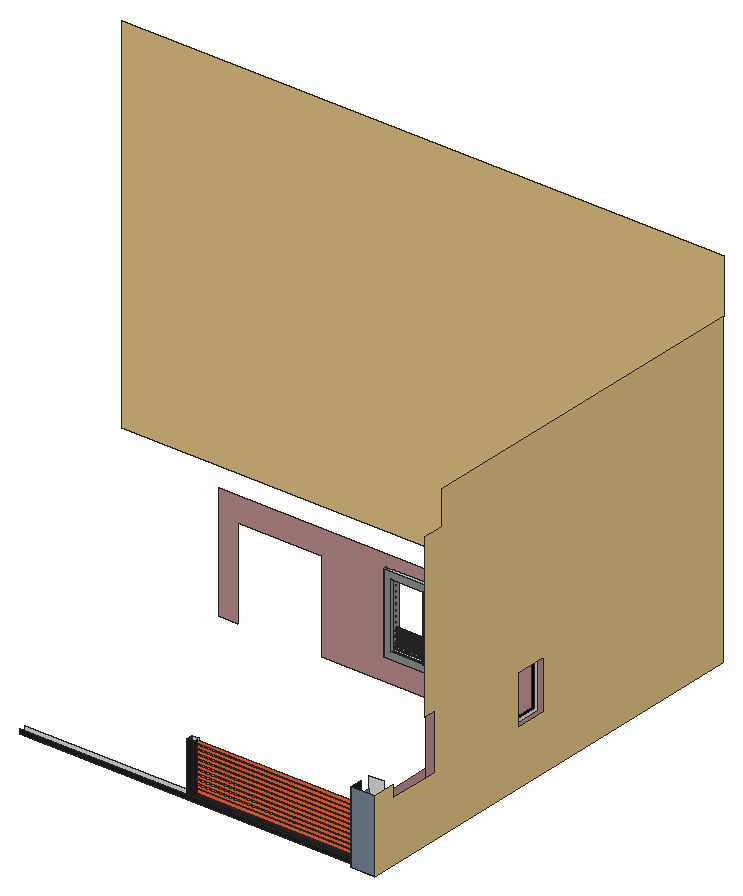
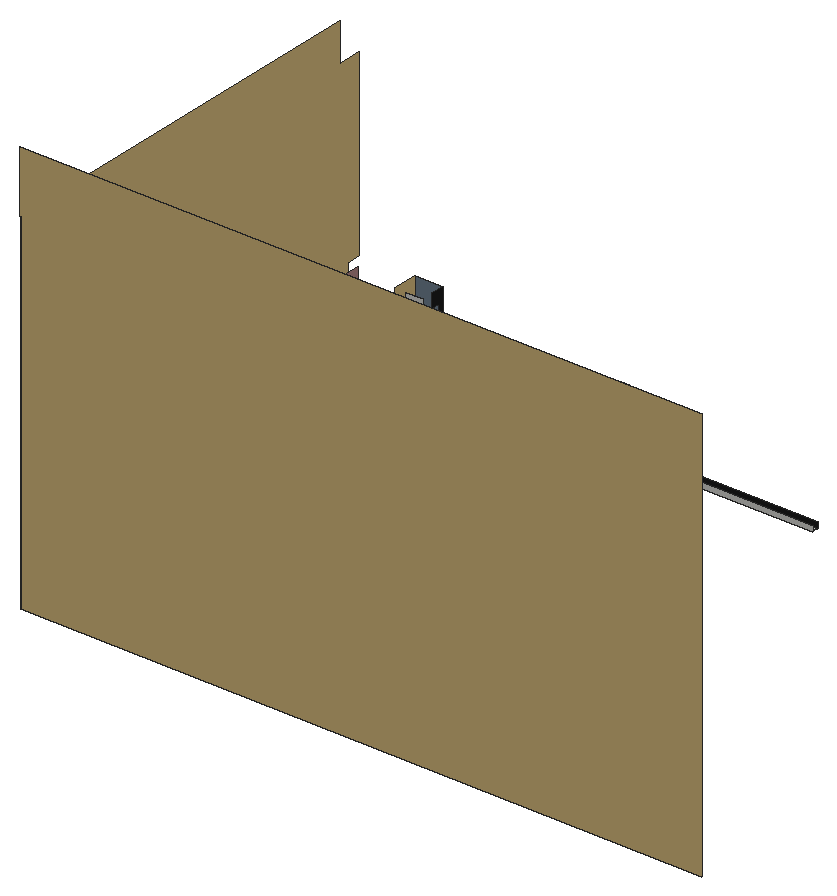
# SketchUp Ruby script. Lengths in inches.
U = 1.inch
M = Sketchup.active_model
def pt(a) = Geom::Point3d.new(a.map { |v| v * U })
def face(e, loops, mat)
  f = e.add_face(loops[0].map { |a| pt(a) })
  loops[1..].each { |l| e.add_face(l.map { |a| pt(a) }).erase! }
  f.material = f.back_material = mat if mat
  f
end
# faces: each face lists its corners as indices into pts; further lists are holes
def faces(e, pts, list, mat = nil) = list.each { |f| face(e, (f[0].is_a?(Array) ? f : [f]).map { |l| l.map { |i| pts[i] } }, mat) }
# xy, xz, yz: faces in a plane at the given z, y or x. An outline is a flat list of corners, or four numbers for a rectangle; further outlines are holes
def ring(l) = l.size == 4 ? [[l[0], l[1]], [l[2], l[1]], [l[2], l[3]], [l[0], l[3]]] : l.each_slice(2).to_a
def flat(e, list, mat, &to3) = list.each { |f| face(e, (f[0].is_a?(Array) ? f : [f]).map { |l| ring(l).map { |u, v| to3.(u, v) } }, mat) }
def xy(e, z, list, mat = nil) = flat(e, list, mat) { |x, y| [x, y, z] }
def xz(e, y, list, mat = nil) = flat(e, list, mat) { |x, z| [x, y, z] }
def yz(e, x, list, mat = nil) = flat(e, list, mat) { |y, z| [x, y, z] }
def lines(e, pts, list) = list.each { |a, b| e.add_line(pt(pts[a]), pt(pts[b])) }
# prism: a flat outline (further loops are holes) pulled along v
def prism(e, loops, v, mat = nil)
  f = face(e, loops, mat); d = Geom::Vector3d.new(v.map { |x| x * U })
  f.pushpull(f.normal.samedirection?(d) ? d.length : -d.length)
end
def box(e, o, s, mat = nil) = prism(e, [[o, [o[0] + s[0], o[1], o[2]], [o[0] + s[0], o[1] + s[1], o[2]], [o[0], o[1] + s[1], o[2]]]], [0, 0, s[2]], mat)
def at(x, y, z, deg = 0) = Geom::Transformation.translation(pt([x, y, z])) * Geom::Transformation.rotation(ORIGIN, Z_AXIS, deg.degrees)
def axes(o, x, y, z) = Geom::Transformation.new([*x, 0, *y, 0, *z, 0, *pt(o).to_a, 1])
def part(name) = M.definitions.add(name)
# library, detail: a bought-in or finely detailed component or shape, given as its bounding box
def library(name, o, s) = part(name).tap { |d| box(d.entities, o, s) }
def detail(e, o, s) = box(e.add_group.entities, o, s)
def put(e, d, t, mat = nil) = e.add_instance(d, t).tap { |i| i.material = mat if mat }
def group(e, t, mat = nil) = e.add_group.tap { |g| g.transformation = t; g.material = mat if mat }.entities
root = M.entities
M.materials.add("[0110_LightSlateGray]").color = [119, 136, 153]
M.materials.add("[0119_RosyBrown]").color = [188, 143, 143]
M.materials.add("[Blacktop Old 02]").color = [143, 145, 145]
M.materials.add("[Color B04]").color = [255, 101, 50]
M.materials.add("[Color M08]").color = [30, 30, 30]
M.materials.add("[Color M09]").color = [0, 0, 0]
M.materials.add("[Concrete Aggregate Smoke]").color = [154, 150, 148]
M.materials.add("[Stone Brushed Khaki]").color = [226, 197, 133]
M.materials.add("[Wood Lumber ButtJoined]").color = [164, 152, 112]
xy(root,0,[[587.78,0,587.78,22.38,602.49,22.38,602.49,74.42,612,74.42,612,0],[254.58,3.88,587.78,6.88],[254.58,6.88,587.78,9.88],[603,74.42,612,135.46],[603,135.46,612,145.85]])
xy(root,4.99,[[421.18,3.88,428.27,6.88],[421.18,6.88,428.27,9.88],[428.27,6.88,587.78,9.88]])
xy(root,4.99,[[428.27,3.88,587.78,6.88]],"[Color M08]")
xy(root,5.875,[[428.27,6.88,587.78,9.88]],"[Color B04]")
xy(root,7.15,[[428.27,6.88,587.78,9.88]],"[Color B04]")
xy(root,10.3125,[[428.27,6.88,587.78,9.88]],"[Color B04]")
xy(root,11.59,[[428.27,6.88,587.78,9.88]],"[Color B04]")
xy(root,14.75,[[428.27,6.88,587.78,9.88]],"[Color B04]")
xy(root,16.03,[[428.27,6.88,587.78,9.88]],"[Color B04]")
xy(root,19.1875,[[428.27,6.88,587.78,9.88]],"[Color B04]")
xy(root,20.46,[[428.27,9.82,587.78,9.88],[428.27,9.88,587.78,9.95],[428.27,9.95,587.78,10.01],[428.27,10.01,587.78,10.13]])
xy(root,20.46,[[428.27,6.88,587.78,9.82]],"[Color B04]")
xy(root,23.35,[[425.53,244.17,512.22,247.17]])
xy(root,23.625,[[428.27,9.82,587.78,9.88],[428.27,9.88,587.78,9.95],[428.27,9.95,587.78,10.01],[428.27,10.01,587.78,10.13]])
xy(root,23.625,[[428.27,6.88,587.78,9.82]],"[Color B04]")
xy(root,24.9,[[428.27,6.88,587.78,9.88]],"[Color B04]")
xy(root,28.0625,[[428.27,6.88,587.78,9.88]],"[Color B04]")
xy(root,29.34,[[428.27,6.88,587.78,9.88]],"[Color B04]")
xy(root,30.2,[[432.38,244.17,464.5,247.17],[464.5,244.17,468.88,247.17],[468.88,244.17,505.38,247.17],[432.38,247.17,464.5,254.42],[468.88,247.17,505.38,254.42]])
xy(root,32.5,[[428.27,6.88,587.78,9.88]],"[Color B04]")
xy(root,33.78,[[428.27,6.88,587.78,9.88]],"[Color B04]")
xy(root,36.9375,[[428.27,6.88,587.78,9.88]],"[Color B04]")
xy(root,38.21,[[428.27,9.88,587.78,10.32]])
xy(root,38.21,[[428.27,6.88,587.78,9.88]],"[Color B04]")
xy(root,41.375,[[428.27,9.88,587.78,10.32]])
xy(root,41.375,[[428.27,6.88,587.78,9.88]],"[Color B04]")
xy(root,42.65,[[428.27,6.88,587.78,9.88]],"[Color B04]")
xy(root,45.8125,[[428.27,6.88,587.78,9.88]],"[Color B04]")
xy(root,47.09,[[428.27,6.88,587.78,9.88]],"[Color B04]")
xy(root,50.25,[[428.27,6.88,587.78,9.88]],"[Color B04]")
xy(root,50.59,[[600,174.3,603,214.68]])
xy(root,51.53,[[428.27,6.88,587.78,9.88]],"[Color B04]")
xz(root,0,[[587.78,0,612,72]],"[0110_LightSlateGray]")
xz(root,3.88,[[254.58,0,587.78,4.99],[421.18,4.99,428.27,54.6875]],"[Color M08]")
xz(root,6.88,[[428.27,4.99,587.78,5.875],[428.27,7.15,587.78,10.3125],[428.27,11.59,587.78,14.75],[428.27,16.03,587.78,19.1875],[428.27,20.46,587.78,23.625],
  [428.27,24.9,587.78,28.0625],[428.27,29.34,587.78,32.5],[428.27,33.78,587.78,36.9375],[428.27,38.21,587.78,41.375],[428.27,42.65,587.78,45.8125],
  [428.27,47.09,587.78,50.25],[428.27,51.53,587.78,54.6875]],"[Color B04]")
xz(root,9.82,[[428.27,20.46,587.78,23.625]])
xz(root,9.88,[[254.58,0,254.58,4.99,428.27,4.99,428.27,2.71,587.78,2.71,587.78,1.4375,428.27,1.4375,428.27,0],[428.27,0,587.78,1.4375],[428.27,2.71,587.78,4.99],[421.18,4.99,428.27,54.6875],[428.27,4.99,587.78,5.875],
  [417.81,6.88,420.87,9],[428.27,7.15,587.78,10.3125],[428.27,11.59,587.78,14.75],[428.27,16.03,587.78,19.1875],[428.27,20.46,587.78,23.625],
  [428.27,24.9,587.78,28.0625],[428.27,29.34,587.78,32.5],[428.27,33.78,587.78,36.9375],[428.27,38.21,587.78,41.375],[428.27,42.65,587.78,45.8125],
  [428.27,47.09,587.78,50.25]])
xz(root,9.88,[[428.27,5.875,587.78,7.15],[428.27,10.3125,587.78,11.59],[428.27,14.75,587.78,16.03],[428.27,19.1875,587.78,20.46],[428.27,23.625,587.78,24.9],
  [428.27,28.0625,587.78,29.34],[428.27,32.5,587.78,33.78],[428.27,36.9375,587.78,38.21],[428.27,41.375,587.78,42.65],[428.27,45.8125,587.78,47.09],
  [428.27,50.25,587.78,51.53]],"[Color B04]")
xz(root,9.95,[[428.27,20.46,587.78,23.625]])
xz(root,10.01,[[428.27,20.46,587.78,23.625]])
xz(root,10.13,[[428.27,20.46,587.78,23.625]])
xz(root,10.32,[[428.27,38.21,587.78,41.375]])
xz(root,22.38,[[587.78,0,602.49,72]])
xz(root,74.42,[[602.49,0,603,60]])
xz(root,174.3,[[600,50.59,603,107.78]],"[Color M09]")
xz(root,214.68,[[600,50.59,603,107.78]])
xz(root,244.17,[[[425.53,23.35,512.22,102.79],[432.38,30.2,505.38,95.95]]],"[Blacktop Old 02]")
xz(root,244.17,[[464.5,30.2,468.88,95.95]],"[Concrete Aggregate Smoke]")
xz(root,247.17,[[[425.53,23.35,512.22,102.79],[432.38,30.2,505.38,95.95]]])
xz(root,247.17,[[[258.19,0,276.99,0,276.99,90.23,361.45,90.23,361.45,0,603,0,603,115.0625,566.2,115.0625,566.2,120,557.23,120,557.23,115.0625,515.23,115.0625,515.23,120,511.18,120,511.18,115.0625,473.23,115.0625,473.23,120,464.26,120,464.26,115.0625,258.19,115.0625],[425.53,23.35,512.22,102.79]]],"[0119_RosyBrown]")
xz(root,434.42,[[12,0,12,364.4375,612.4375,364.4375,612.4375,310.0625,612,310.0625,612,0]],"[Stone Brushed Khaki]")
yz(root,420.87,[[6.88,6.88,9.88,9]])
yz(root,421.18,[[6.88,10.58,9.88,12.6875],[6.88,14.45,9.88,16.5625],[6.88,18.26,9.88,20.375],[6.88,22.08,9.88,24.1875],[6.88,25.89,9.88,28],
  [6.88,29.7,9.88,31.8125],[6.88,33.51,9.88,35.625],[6.88,37.33,9.88,39.4375],[6.88,41.14,9.88,43.25],[6.88,44.95,9.88,47.0625],
  [6.88,48.76,9.88,50.875]])
yz(root,421.18,[[3.88,4.99,3.88,54.6875,6.88,54.6875,6.88,52.58,9.88,52.58,9.88,50.875,6.88,50.875,6.88,48.76,9.88,48.76,9.88,47.0625,6.88,47.0625,6.88,44.95,9.88,44.95,9.88,43.25,6.88,43.25,6.88,41.14,9.88,41.14,9.88,39.4375,6.88,39.4375,6.88,37.33,9.88,37.33,9.88,35.625,6.88,35.625,6.88,33.51,9.88,33.51,9.88,31.8125,6.88,31.8125,6.88,29.7,9.88,29.7,9.88,28,6.88,28,6.88,25.89,9.88,25.89,9.88,24.1875,6.88,24.1875,6.88,22.08,9.88,22.08,9.88,20.375,6.88,20.375,6.88,18.26,9.88,18.26,9.88,16.5625,6.88,16.5625,6.88,14.45,9.88,14.45,9.88,12.6875,6.88,12.6875,6.88,10.58,9.88,10.58,9.88,4.99]],"[Color M08]")
yz(root,425.53,[[244.17,23.35,247.17,102.79]],"[Blacktop Old 02]")
yz(root,428.27,[[6.88,4.99,9.88,5.875],[6.88,7.15,9.88,10.3125],[6.88,11.59,9.88,14.75],[6.88,16.03,9.88,19.1875],[6.88,20.46,9.82,23.625],
  [9.82,20.46,9.88,23.625],[9.88,20.46,9.95,23.625],[9.95,20.46,10.01,23.625],[10.01,20.46,10.13,23.625],[6.88,24.9,9.88,28.0625],
  [6.88,29.34,9.88,32.5],[6.88,33.78,9.88,36.9375],[6.88,38.21,9.88,41.375],[9.88,38.21,10.32,41.375],[6.88,42.65,9.88,45.8125],
  [6.88,47.09,9.88,50.25],[6.88,51.53,9.88,54.6875]])
yz(root,428.27,[[3.88,4.99,6.88,4.99,6.88,5.875,9.88,5.875,9.88,7.15,6.88,7.15,6.88,10.3125,9.88,10.3125,9.88,11.59,6.88,11.59,6.88,14.75,9.88,14.75,9.88,16.03,6.88,16.03,6.88,19.1875,9.88,19.1875,9.88,20.46,6.88,20.46,6.88,23.625,9.88,23.625,9.88,24.9,6.88,24.9,6.88,28.0625,9.88,28.0625,9.88,29.34,6.88,29.34,6.88,32.5,9.88,32.5,9.88,33.78,6.88,33.78,6.88,36.9375,9.88,36.9375,9.88,38.21,6.88,38.21,6.88,41.375,9.88,41.375,9.88,42.65,6.88,42.65,6.88,45.8125,9.88,45.8125,9.88,47.09,6.88,47.09,6.88,50.25,9.88,50.25,9.88,51.53,6.88,51.53,6.88,54.6875,3.88,54.6875]],"[Color M08]")
yz(root,432.38,[[244.17,30.2,247.17,95.95],[[247.17,30.2,254.42,95.95],[250.66,85.64,250.21,85.7,249.78,85.88,249.42,86.16,249.14,86.52,248.97,86.94,248.91,87.39,248.97,87.85,249.14,88.27,249.42,88.63,249.78,88.91,250.21,89.09,250.66,89.14,251.11,89.09,251.53,88.91,251.9,88.63,252.18,88.27,252.35,87.85,252.41,87.39,252.35,86.94,252.18,86.52,251.9,86.16,251.53,85.88,251.11,85.7],[250.66,80.08,250.21,80.14,249.78,80.32,249.42,80.59,249.14,80.96,248.97,81.38,248.91,81.83,248.97,82.29,249.14,82.71,249.42,83.07,249.78,83.35,250.21,83.52,250.66,83.58,251.11,83.52,251.53,83.35,251.9,83.07,252.18,82.71,252.35,82.29,252.41,81.83,252.35,81.38,252.18,80.96,251.9,80.59,251.53,80.32,251.11,80.14],[250.66,74.52,250.21,74.58,249.78,74.75,249.42,75.03,249.14,75.39,248.97,75.82,248.91,76.27,248.97,76.72,249.14,77.14,249.42,77.51,249.78,77.79,250.21,77.96,250.66,78.02,251.11,77.96,251.53,77.79,251.9,77.51,252.18,77.14,252.35,76.72,252.41,76.27,252.35,75.82,252.18,75.39,251.9,75.03,251.53,74.75,251.11,74.58],[250.66,68.96,250.21,69.02,249.78,69.19,249.42,69.47,249.14,69.83,248.97,70.25,248.91,70.71,248.97,71.16,249.14,71.58,249.42,71.94,249.78,72.22,250.21,72.4,250.66,72.46,251.11,72.4,251.53,72.22,251.9,71.94,252.18,71.58,252.35,71.16,252.41,70.71,252.35,70.25,252.18,69.83,251.9,69.47,251.53,69.19,251.11,69.02],[250.66,63.39,250.21,63.45,249.78,63.63,249.42,63.91,249.14,64.27,248.97,64.69,248.91,65.14,248.97,65.6,249.14,66.02,249.42,66.38,249.78,66.66,250.21,66.84,250.66,66.89,251.11,66.84,251.53,66.66,251.9,66.38,252.18,66.02,252.35,65.6,252.41,65.14,252.35,64.69,252.18,64.27,251.9,63.91,251.53,63.63,251.11,63.45],[250.66,57.83,250.21,57.89,249.78,58.07,249.42,58.34,249.14,58.71,248.97,59.13,248.91,59.58,248.97,60.04,249.14,60.46,249.42,60.82,249.78,61.1,250.21,61.27,250.66,61.33,251.11,61.27,251.53,61.1,251.9,60.82,252.18,60.46,252.35,60.04,252.41,59.58,252.35,59.13,252.18,58.71,251.9,58.34,251.53,58.07,251.11,57.89],[250.66,52.27,250.21,52.33,249.78,52.5,249.42,52.78,249.14,53.14,248.97,53.57,248.91,54.02,248.97,54.47,249.14,54.89,249.42,55.26,249.78,55.54,250.21,55.71,250.66,55.77,251.11,55.71,251.53,55.54,251.9,55.26,252.18,54.89,252.35,54.47,252.41,54.02,252.35,53.57,252.18,53.14,251.9,52.78,251.53,52.5,251.11,52.33],[250.66,46.71,250.21,46.77,249.78,46.94,249.42,47.22,249.14,47.58,248.97,48,248.91,48.46,248.97,48.91,249.14,49.33,249.42,49.69,249.78,49.97,250.21,50.15,250.66,50.21,251.11,50.15,251.53,49.97,251.9,49.69,252.18,49.33,252.35,48.91,252.41,48.46,252.35,48,252.18,47.58,251.9,47.22,251.53,46.94,251.11,46.77],[250.66,41.14,250.21,41.2,249.78,41.38,249.42,41.66,249.14,42.02,248.97,42.44,248.91,42.89,248.97,43.35,249.14,43.77,249.42,44.13,249.78,44.41,250.21,44.59,250.66,44.64,251.11,44.59,251.53,44.41,251.9,44.13,252.18,43.77,252.35,43.35,252.41,42.89,252.35,42.44,252.18,42.02,251.9,41.66,251.53,41.38,251.11,41.2],[250.66,35.58,250.21,35.64,249.78,35.82,249.42,36.09,249.14,36.46,248.97,36.88,248.91,37.33,248.97,37.79,249.14,38.21,249.42,38.57,249.78,38.85,250.21,39.02,250.66,39.08,251.11,39.02,251.53,38.85,251.9,38.57,252.18,38.21,252.35,37.79,252.41,37.33,252.35,36.88,252.18,36.46,251.9,36.09,251.53,35.82,251.11,35.64],[250.66,91.21,250.21,91.27,249.78,91.44,249.42,91.72,249.14,92.08,248.97,92.5,248.91,92.96,248.97,93.41,249.14,93.83,249.42,94.19,249.78,94.47,250.21,94.65,250.66,94.71,251.11,94.65,251.53,94.47,251.9,94.19,252.18,93.83,252.35,93.41,252.41,92.96,252.35,92.5,252.18,92.08,251.9,91.72,251.53,91.44,251.11,91.27]]],"[Blacktop Old 02]")
yz(root,464.5,[[244.17,30.2,254.42,95.95]],"[Concrete Aggregate Smoke]")
yz(root,468.88,[[244.17,30.2,254.42,95.95]],"[Concrete Aggregate Smoke]")
yz(root,504.69,[[250.66,35.58,251.11,35.64,251.53,35.82,251.9,36.09,252.18,36.46,252.35,36.88,252.41,37.33,252.35,37.79,252.18,38.21,251.9,38.57,251.53,38.85,251.11,39.02,250.66,39.08,250.21,39.02,249.78,38.85,249.42,38.57,249.14,38.21,248.97,37.79,248.91,37.33,248.97,36.88,249.14,36.46,249.42,36.09,249.78,35.82,250.21,35.64]])
yz(root,505.38,[[244.17,30.2,247.17,95.95],[[247.17,30.2,254.42,95.95],[250.66,85.64,251.11,85.7,251.53,85.88,251.9,86.16,252.18,86.52,252.35,86.94,252.41,87.39,252.35,87.85,252.18,88.27,251.9,88.63,251.53,88.91,251.11,89.09,250.66,89.14,250.21,89.09,249.78,88.91,249.42,88.63,249.14,88.27,248.97,87.85,248.91,87.39,248.97,86.94,249.14,86.52,249.42,86.16,249.78,85.88,250.21,85.7],[250.66,80.08,251.11,80.14,251.53,80.32,251.9,80.59,252.18,80.96,252.35,81.38,252.41,81.83,252.35,82.29,252.18,82.71,251.9,83.07,251.53,83.35,251.11,83.52,250.66,83.58,250.21,83.52,249.78,83.35,249.42,83.07,249.14,82.71,248.97,82.29,248.91,81.83,248.97,81.38,249.14,80.96,249.42,80.59,249.78,80.32,250.21,80.14],[250.66,74.52,251.11,74.58,251.53,74.75,251.9,75.03,252.18,75.39,252.35,75.82,252.41,76.27,252.35,76.72,252.18,77.14,251.9,77.51,251.53,77.79,251.11,77.96,250.66,78.02,250.21,77.96,249.78,77.79,249.42,77.51,249.14,77.14,248.97,76.72,248.91,76.27,248.97,75.82,249.14,75.39,249.42,75.03,249.78,74.75,250.21,74.58],[250.66,68.96,251.11,69.02,251.53,69.19,251.9,69.47,252.18,69.83,252.35,70.25,252.41,70.71,252.35,71.16,252.18,71.58,251.9,71.94,251.53,72.22,251.11,72.4,250.66,72.46,250.21,72.4,249.78,72.22,249.42,71.94,249.14,71.58,248.97,71.16,248.91,70.71,248.97,70.25,249.14,69.83,249.42,69.47,249.78,69.19,250.21,69.02],[250.66,63.39,251.11,63.45,251.53,63.63,251.9,63.91,252.18,64.27,252.35,64.69,252.41,65.14,252.35,65.6,252.18,66.02,251.9,66.38,251.53,66.66,251.11,66.84,250.66,66.89,250.21,66.84,249.78,66.66,249.42,66.38,249.14,66.02,248.97,65.6,248.91,65.14,248.97,64.69,249.14,64.27,249.42,63.91,249.78,63.63,250.21,63.45],[250.66,57.83,251.11,57.89,251.53,58.07,251.9,58.34,252.18,58.71,252.35,59.13,252.41,59.58,252.35,60.04,252.18,60.46,251.9,60.82,251.53,61.1,251.11,61.27,250.66,61.33,250.21,61.27,249.78,61.1,249.42,60.82,249.14,60.46,248.97,60.04,248.91,59.58,248.97,59.13,249.14,58.71,249.42,58.34,249.78,58.07,250.21,57.89],[250.66,52.27,251.11,52.33,251.53,52.5,251.9,52.78,252.18,53.14,252.35,53.57,252.41,54.02,252.35,54.47,252.18,54.89,251.9,55.26,251.53,55.54,251.11,55.71,250.66,55.77,250.21,55.71,249.78,55.54,249.42,55.26,249.14,54.89,248.97,54.47,248.91,54.02,248.97,53.57,249.14,53.14,249.42,52.78,249.78,52.5,250.21,52.33],[250.66,41.14,251.11,41.2,251.53,41.38,251.9,41.66,252.18,42.02,252.35,42.44,252.41,42.89,252.35,43.35,252.18,43.77,251.9,44.13,251.53,44.41,251.11,44.59,250.66,44.64,250.21,44.59,249.78,44.41,249.42,44.13,249.14,43.77,248.97,43.35,248.91,42.89,248.97,42.44,249.14,42.02,249.42,41.66,249.78,41.38,250.21,41.2]]],"[Blacktop Old 02]")
yz(root,506.44,[[250.66,46.71,251.11,46.77,251.53,46.94,251.9,47.22,252.18,47.58,252.35,48,252.41,48.46,252.35,48.91,252.18,49.33,251.9,49.69,251.53,49.97,251.11,50.15,250.66,50.21,250.21,50.15,249.78,49.97,249.42,49.69,249.14,49.33,248.97,48.91,248.91,48.46,248.97,48,249.14,47.58,249.42,47.22,249.78,46.94,250.21,46.77]])
yz(root,512.22,[[244.17,23.35,247.17,102.79]],"[Blacktop Old 02]")
yz(root,587.78,[[3.88,0,6.88,4.99],[6.88,0,9.88,4.99],[6.88,4.99,9.88,5.875],[6.88,7.15,9.88,10.3125],[6.88,11.59,9.88,14.75],
  [6.88,16.03,9.88,19.1875],[6.88,20.46,9.82,23.625],[9.82,20.46,9.88,23.625],[9.88,20.46,9.95,23.625],[9.95,20.46,10.01,23.625],
  [10.01,20.46,10.13,23.625],[6.88,24.9,9.88,28.0625],[6.88,29.34,9.88,32.5],[6.88,33.78,9.88,36.9375],[6.88,38.21,9.88,41.375],
  [9.88,38.21,10.32,41.375],[6.88,42.65,9.88,45.8125],[6.88,47.09,9.88,50.25]])
yz(root,587.78,[[9.88,0,9.88,20.46,10.13,20.46,10.13,23.625,9.88,23.625,9.88,38.21,10.32,38.21,10.32,41.375,9.88,41.375,9.88,51.53,6.88,51.53,6.88,54.6875,9.88,54.6875,9.88,60,22.38,60,22.38,0]],"[0110_LightSlateGray]")
yz(root,587.78,[[0,0,0,72,12,72,12,60,3.88,60,3.88,54.6875,6.88,54.6875,6.88,51.53,9.88,51.53,9.88,50.25,6.88,50.25,6.88,47.09,9.88,47.09,9.88,45.8125,6.88,45.8125,6.88,42.65,9.88,42.65,9.88,41.375,6.88,41.375,6.88,38.21,9.88,38.21,9.88,36.9375,6.88,36.9375,6.88,33.78,9.88,33.78,9.88,32.5,6.88,32.5,6.88,29.34,9.88,29.34,9.88,28.0625,6.88,28.0625,6.88,24.9,9.88,24.9,9.88,23.625,6.88,23.625,6.88,20.46,9.88,20.46,9.88,19.1875,6.88,19.1875,6.88,16.03,9.88,16.03,9.88,14.75,6.88,14.75,6.88,11.59,9.88,11.59,9.88,10.3125,6.88,10.3125,6.88,7.15,9.88,7.15,9.88,5.875,6.88,5.875,6.88,4.99,3.88,4.99,3.88,0]],"[Color M08]")
yz(root,600,[[[174.3,50.59,214.68,107.78],[178.05,54.34,210.93,104.03]]],"[Color M09]")
yz(root,602.49,[[22.38,0,74.42,60]],"[0119_RosyBrown]")
yz(root,603,[[254.42,0,425.42,120],[[174.3,50.59,214.68,107.78],[178.05,54.34,210.93,104.03]]])
yz(root,603,[[[74.42,0,247.17,115.0625],[174.3,50.59,214.68,107.78]]],"[0119_RosyBrown]")
yz(root,612,[[[0,0,434.42,0,434.42,310.0625,83.42,310.0625,83.42,276,62.42,276,62.42,115.0625,74.42,115.0625,74.42,60,22.38,60,22.38,72,0,72],[178.05,54.34,210.93,104.03]]],"[Stone Brushed Khaki]")
p = [[432.38,248.47,31.51],[432.38,248.92,31.45],[504.69,248.92,31.45],[504.69,248.47,31.51],[432.38,249.375,31.51],[504.69,249.375,31.51],
  [432.38,248.05,31.68],[504.69,248.05,31.68],[432.38,249.8,31.68],[504.69,249.8,31.68],[432.38,247.68,31.96],[504.69,247.68,31.96],
  [432.38,250.16,31.96],[504.69,250.16,31.96],[432.38,247.4,32.32],[504.69,247.4,32.32],[432.38,250.4375,32.32],[504.69,250.4375,32.32],
  [432.38,247.23,32.75],[504.69,247.23,32.75],[432.38,250.61,32.75],[504.69,250.61,32.75],[432.38,247.17,33.2],[504.69,247.17,33.2],
  [432.38,250.67,33.2],[504.69,250.67,33.2],[432.38,247.23,33.65],[504.69,247.23,33.65],[432.38,250.61,33.65],[504.69,250.61,33.65],
  [432.38,247.4,34.07],[504.69,247.4,34.07],[432.38,250.4375,34.07],[504.69,250.4375,34.07],[432.38,247.68,34.4375],[504.69,247.68,34.4375],
  [432.38,250.16,34.4375],[504.69,250.16,34.4375],[432.38,248.05,34.71],[504.69,248.05,34.71],[432.38,249.8,34.71],[504.69,249.8,34.71],
  [432.38,248.47,34.89],[504.69,248.47,34.89],[432.38,249.375,34.89],[504.69,249.375,34.89],[432.38,248.92,34.95],[504.69,248.92,34.95],
  [432.38,249.78,35.82],[432.38,250.21,35.64],[504.69,250.21,35.64],[504.69,249.78,35.82],[432.38,250.66,35.58],[504.69,250.66,35.58],
  [432.38,251.11,35.64],[504.69,251.11,35.64],[432.38,251.53,35.82],[504.69,251.53,35.82],[432.38,249.42,36.09],[504.69,249.42,36.09],
  [432.38,251.9,36.09],[504.69,251.9,36.09],[432.38,249.14,36.46],[504.69,249.14,36.46],[432.38,252.18,36.46],[504.69,252.18,36.46],
  [432.38,248.97,36.88],[504.69,248.97,36.88],[432.38,252.35,36.88],[504.69,252.35,36.88],[432.38,248.91,37.33],[504.69,248.91,37.33],
  [432.38,252.41,37.33],[504.69,252.41,37.33],[432.38,248.97,37.79],[504.69,248.97,37.79],[432.38,252.35,37.79],[504.69,252.35,37.79],
  [432.38,249.14,38.21],[504.69,249.14,38.21],[432.38,252.18,38.21],[504.69,252.18,38.21],[432.38,249.42,38.57],[504.69,249.42,38.57],
  [432.38,251.9,38.57],[504.69,251.9,38.57],[432.38,249.78,38.85],[504.69,249.78,38.85],[432.38,251.53,38.85],[504.69,251.53,38.85],
  [432.38,250.21,39.02],[504.69,250.21,39.02],[432.38,251.11,39.02],[504.69,251.11,39.02],[432.38,250.66,39.08],[504.69,250.66,39.08],
  [432.38,250.21,41.2],[432.38,250.66,41.14],[505.38,250.66,41.14],[505.38,250.21,41.2],[432.38,251.11,41.2],[505.38,251.11,41.2],
  [432.38,249.78,41.38],[505.38,249.78,41.38],[432.38,251.53,41.38],[505.38,251.53,41.38],[432.38,249.42,41.66],[505.38,249.42,41.66],
  [432.38,251.9,41.66],[505.38,251.9,41.66],[432.38,249.14,42.02],[505.38,249.14,42.02],[432.38,252.18,42.02],[505.38,252.18,42.02],
  [432.38,248.97,42.44],[505.38,248.97,42.44],[432.38,252.35,42.44],[505.38,252.35,42.44],[432.38,248.91,42.89],[505.38,248.91,42.89],
  [432.38,252.41,42.89],[505.38,252.41,42.89],[432.38,248.97,43.35],[505.38,248.97,43.35],[432.38,252.35,43.35],[505.38,252.35,43.35],
  [432.38,249.14,43.77],[505.38,249.14,43.77],[432.38,252.18,43.77],[505.38,252.18,43.77],[432.38,249.42,44.13],[505.38,249.42,44.13],
  [432.38,251.9,44.13],[505.38,251.9,44.13],[432.38,249.78,44.41],[505.38,249.78,44.41],[432.38,251.53,44.41],[505.38,251.53,44.41],
  [432.38,250.21,44.59],[505.38,250.21,44.59],[432.38,251.11,44.59],[505.38,251.11,44.59],[432.38,250.66,44.64],[505.38,250.66,44.64],
  [432.38,250.21,46.77],[432.38,250.66,46.71],[506.44,250.66,46.71],[506.44,250.21,46.77],[432.38,251.11,46.77],[506.44,251.11,46.77],
  [432.38,249.78,46.94],[506.44,249.78,46.94],[432.38,251.53,46.94],[506.44,251.53,46.94],[432.38,249.42,47.22],[506.44,249.42,47.22],
  [432.38,251.9,47.22],[506.44,251.9,47.22],[432.38,249.14,47.58],[506.44,249.14,47.58],[432.38,252.18,47.58],[506.44,252.18,47.58],
  [432.38,248.97,48],[506.44,248.97,48],[432.38,252.35,48],[506.44,252.35,48],[432.38,248.91,48.46],[506.44,248.91,48.46],
  [432.38,252.41,48.46],[506.44,252.41,48.46],[432.38,248.97,48.91],[506.44,248.97,48.91],[432.38,252.35,48.91],[506.44,252.35,48.91],
  [432.38,249.14,49.33],[506.44,249.14,49.33],[432.38,252.18,49.33],[506.44,252.18,49.33],[432.38,249.42,49.69],[506.44,249.42,49.69],
  [432.38,251.9,49.69],[506.44,251.9,49.69],[432.38,249.78,49.97],[506.44,249.78,49.97],[432.38,251.53,49.97],[506.44,251.53,49.97],
  [432.38,250.21,50.15],[506.44,250.21,50.15],[432.38,251.11,50.15],[506.44,251.11,50.15],[432.38,250.66,50.21],[506.44,250.66,50.21],
  [587.78,9.88,-1.72],[587.78,9.88,0]]
faces(root,p,[[0,1,2,3],[1,4,5,2],[6,0,3,7],[4,8,9,5],[10,6,7,11],[8,12,13,9],[14,10,11,15],[12,16,17,13],
  [18,14,15,19],[16,20,21,17],[22,18,19,23],[20,24,25,21],[26,22,23,27],[24,28,29,25],[30,26,27,31],[28,32,33,29],
  [34,30,31,35],[32,36,37,33],[38,34,35,39],[36,40,41,37],[42,38,39,43],[40,44,45,41],[46,42,43,47],[44,46,47,45],
  [48,49,50,51],[49,52,53,50],[52,54,55,53],[54,56,57,55],[58,48,51,59],[56,60,61,57],[62,58,59,63],[60,64,65,61],
  [66,62,63,67],[64,68,69,65],[70,66,67,71],[68,72,73,69],[74,70,71,75],[72,76,77,73],[78,74,75,79],[76,80,81,77],
  [82,78,79,83],[80,84,85,81],[86,82,83,87],[84,88,89,85],[90,86,87,91],[88,92,93,89],[94,90,91,95],[92,94,95,93],
  [96,97,98,99],[97,100,101,98],[102,96,99,103],[100,104,105,101],[106,102,103,107],[104,108,109,105],[110,106,107,111],[108,112,113,109],
  [114,110,111,115],[112,116,117,113],[118,114,115,119],[116,120,121,117],[122,118,119,123],[120,124,125,121],[126,122,123,127],[124,128,129,125],
  [130,126,127,131],[128,132,133,129],[134,130,131,135],[132,136,137,133],[138,134,135,139],[136,140,141,137],[142,138,139,143],[140,142,143,141],
  [144,145,146,147],[145,148,149,146],[150,144,147,151],[148,152,153,149],[154,150,151,155],[152,156,157,153],[158,154,155,159],[156,160,161,157],
  [162,158,159,163],[160,164,165,161],[166,162,163,167],[164,168,169,165],[170,166,167,171],[168,172,173,169],[174,170,171,175],[172,176,177,173],
  [178,174,175,179],[176,180,181,177],[182,178,179,183],[180,184,185,181],[186,182,183,187],[184,188,189,185],[190,186,187,191],[188,190,191,189]],"[Wood Lumber ButtJoined]")
lines(root,p,[[192,193]])
